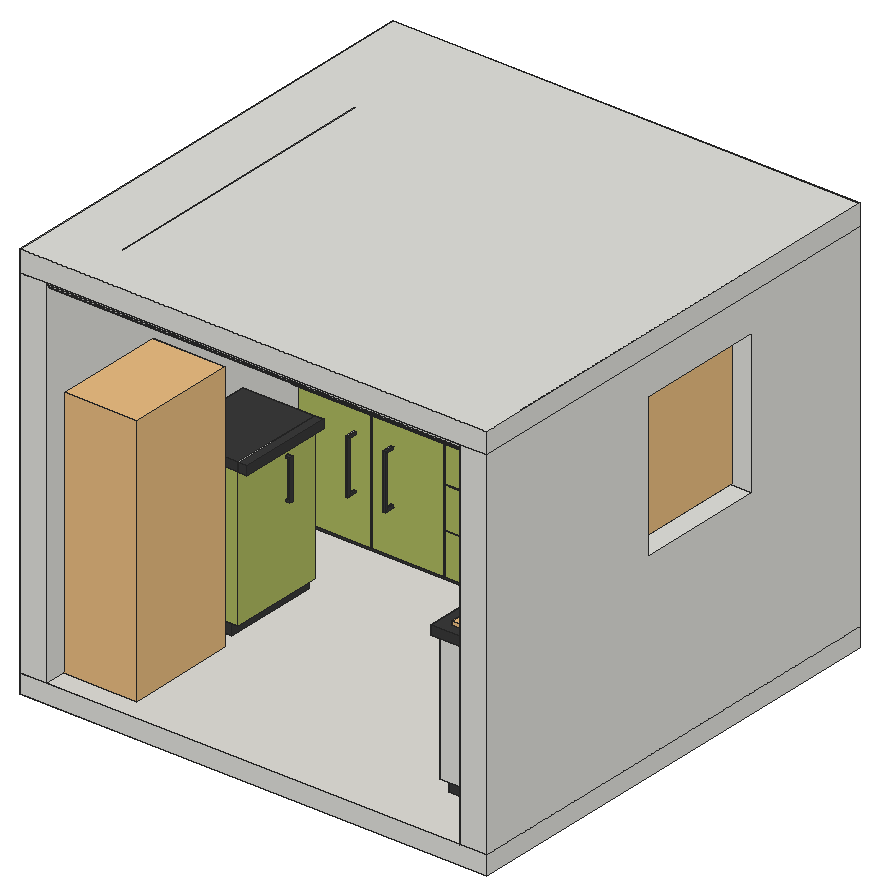
# SketchUp Ruby script. Lengths in inches.
U = 1.inch
M = Sketchup.active_model
def pt(a) = Geom::Point3d.new(a.map { |v| v * U })
def face(e, loops, mat)
  f = e.add_face(loops[0].map { |a| pt(a) })
  loops[1..].each { |l| e.add_face(l.map { |a| pt(a) }).erase! }
  f.material = f.back_material = mat if mat
  f
end
# faces: each face lists its corners as indices into pts; further lists are holes
def faces(e, pts, list, mat = nil) = list.each { |f| face(e, (f[0].is_a?(Array) ? f : [f]).map { |l| l.map { |i| pts[i] } }, mat) }
# xy, xz, yz: faces in a plane at the given z, y or x. An outline is a flat list of corners, or four numbers for a rectangle; further outlines are holes
def ring(l) = l.size == 4 ? [[l[0], l[1]], [l[2], l[1]], [l[2], l[3]], [l[0], l[3]]] : l.each_slice(2).to_a
def flat(e, list, mat, &to3) = list.each { |f| face(e, (f[0].is_a?(Array) ? f : [f]).map { |l| ring(l).map { |u, v| to3.(u, v) } }, mat) }
def xy(e, z, list, mat = nil) = flat(e, list, mat) { |x, y| [x, y, z] }
def xz(e, y, list, mat = nil) = flat(e, list, mat) { |x, z| [x, y, z] }
def yz(e, x, list, mat = nil) = flat(e, list, mat) { |y, z| [x, y, z] }
def lines(e, pts, list) = list.each { |a, b| e.add_line(pt(pts[a]), pt(pts[b])) }
# prism: a flat outline (further loops are holes) pulled along v
def prism(e, loops, v, mat = nil)
  f = face(e, loops, mat); d = Geom::Vector3d.new(v.map { |x| x * U })
  f.pushpull(f.normal.samedirection?(d) ? d.length : -d.length)
end
def box(e, o, s, mat = nil) = prism(e, [[o, [o[0] + s[0], o[1], o[2]], [o[0] + s[0], o[1] + s[1], o[2]], [o[0], o[1] + s[1], o[2]]]], [0, 0, s[2]], mat)
def at(x, y, z, deg = 0) = Geom::Transformation.translation(pt([x, y, z])) * Geom::Transformation.rotation(ORIGIN, Z_AXIS, deg.degrees)
def axes(o, x, y, z) = Geom::Transformation.new([*x, 0, *y, 0, *z, 0, *pt(o).to_a, 1])
def part(name) = M.definitions.add(name)
# library, detail: a bought-in or finely detailed component or shape, given as its bounding box
def library(name, o, s) = part(name).tap { |d| box(d.entities, o, s) }
def detail(e, o, s) = box(e.add_group.entities, o, s)
def put(e, d, t, mat = nil) = e.add_instance(d, t).tap { |i| i.material = mat if mat }
def group(e, t, mat = nil) = e.add_group.tap { |g| g.transformation = t; g.material = mat if mat }.entities
root = M.entities
M.materials.add("Decor - Olives").color = [174, 186, 96]
M.materials.add("[Color_007]").color = [58, 58, 58]
M.materials.add("[Marble Carrara Gold Floor Tile]").color = [225, 223, 217]
M.materials.add("[Tile Limestone Large]").color = [238, 251, 230]
M.materials.add("[Translucent Glass Dark Green]").color = [62, 91, 5]
M.materials["[Translucent Glass Dark Green]"].alpha = 0.5
M.materials.add("besi putih_Glossy3").color = [240, 240, 240]
M.materials.add("go trang").color = [128, 128, 128]
M.materials.add("sink-modena").color = [184, 184, 183]
c1 = library("Chimney (1)",[0,-14.34,0],[33.95,14.34,33.72])
c2 = library("365+Glass+Boxes",[-18.57,-9.91,0],[15.17,6.51,15.85])
c3 = library("FF_ceramic_large_dish_green_FMH",[0,0,0],[11.8125,11.8125,0.53])
c4 = library("FF_ceramic_medium_dish_blue_FMH",[0,0,0],[8.27,8.27,0.53])
c5 = library("FF_dish_rack_plastic_base_03_FMH",[-0.59,0,0],[11.88,20.6,0.91])
c6 = library("FF_dish_rack_cup_FMH\#1",[0,0.11,-0.46],[7.68,3.36,4.07])
c7 = library("FF_dish_rack_03_FMH",[0,0,0],[17.32,9.65,4.94])
c8 = library("FF_ceramic_medium_dish_red_FMH",[0,0,0],[8.27,8.27,0.53])
c9 = library("Kitchen utensil rack",[7.875,0,-1.06],[35.44,4.85,11.83])
c10 = library("kitchen",[57.57,5.21,10.61],[18.31,18.31,13.72])
c11 = library("French glass door with glass lintels",[-8.63,0,-6],[91.05,103.25,8])
c12 = library("Gas+stove+1",[-1.375,6.69,0.47],[35.625,31.32,3.01])
c13 = library("FF_flatware_wood_grip_placed_FMH\#1",[-5.7,-0.44,-1.47],[7.04,11.15,5.13])
c14 = library("Kitchen kettle",[-1.02,0.04,0],[9.81,8.74,8.22])
c15 = library("Drip coffee maker",[0,0,0.5],[20.95,10.01,8.67])
c16 = library("FF_Model_ID12346_3_IlluminatedPlanterCollectionLiscioCF3SU7",[0,0,0],[43.54,41.82,102.67])
c17 = library("itchenFaucet_Handspray\#1",[0.83,4.01,0],[10.6,4,15.3])
c18 = library("Kitchen towel rack",[0,0,-11.5625],[20.09,4.25,16.29])
c19 = library("Untitled (6)",[-101.41,0,-4.6],[35.6,35.6,49.16])
c20 = library("Component\#33",[0,0,0],[60.64,55.48,158.625])
c21 = library("Group\#225",[0,0,0],[3.9375,3.9375,5.51])
c22 = library("Group\#125",[0,0,-0.51],[31.38,18.97,5.43])
xy(root,-6.32,[[0,0,156.125,156.125]])
xy(root,0,[[0,0,0,156.125,156.125,156.125,156.125,0,147.125,0,147.125,20.1875,127.25,20.1875,127.25,108.125,9,108.125,9,81.875,31,81.875,31,50,9,50,9,0]])
xy(root,0,[[9,0,147.125,0,147.125,20.1875,127.25,20.1875,127.25,108.125,9,108.125,9,81.875,31,81.875,31,50,9,50]],"[Marble Carrara Gold Floor Tile]")
xy(root,3,[[124.25,20.1875,127.25,41.12],[124.55,41.12,127.25,41.42],[124.25,41.42,127.25,62.36],[124.55,62.36,127.25,62.66],[124.25,62.66,127.25,83.59],
  [124.55,83.59,127.25,83.89],[124.25,83.89,127.25,105.125],[9,105.125,33.4375,108.125],[33.74,105.125,33.74,105.43,33.4375,105.43,33.4375,108.125,57.875,108.125,57.875,105.125],[58.18,105.125,58.18,105.43,57.875,105.43,57.875,108.125,96.1875,108.125,96.1875,105.125],
  [96.49,105.125,96.49,105.43,96.1875,105.43,96.1875,108.125,127.25,108.125,127.25,105.125]])
xy(root,3.6875,[[9,50,31,81.875],[31,50,33,81.875]])
xy(root,7.66,[[69.52,103.2,69.52,105.125,70.21,105.125,70.21,103.88,79.5625,103.88,79.5625,105.125,80.25,105.125,80.25,103.2]],"[Color_007]")
xy(root,8.22,[[69.52,103.2,80.25,103.2,80.25,105.125,79.5625,105.125,79.5625,103.88,70.21,103.88,70.21,105.125,69.52,105.125]],"[Color_007]")
xy(root,16.7,[[58.18,105.125,96.1875,105.43]])
xy(root,17,[[58.18,105.125,96.1875,105.43]])
xy(root,23.22,[[69.52,103.2,69.52,105.125,70.21,105.125,70.21,103.88,79.5625,103.88,79.5625,105.125,80.25,105.125,80.25,103.2]],"[Color_007]")
xy(root,23.78,[[69.52,103.2,80.25,103.2,80.25,105.125,79.5625,105.125,79.5625,103.88,70.21,103.88,70.21,105.125,69.52,105.125]],"[Color_007]")
xy(root,30.7,[[58.18,105.125,96.1875,105.43]])
xy(root,31,[[58.18,105.125,96.1875,105.43]])
xy(root,38.78,[[69.52,103.2,69.52,105.125,70.21,105.125,70.21,103.88,79.5625,103.88,79.5625,105.125,80.25,105.125,80.25,103.2]],"[Color_007]")
xy(root,39.34,[[69.52,103.2,80.25,103.2,80.25,105.125,79.5625,105.125,79.5625,103.88,70.21,103.88,70.21,105.125,69.52,105.125]],"[Color_007]")
xy(root,41.75,[[127.45,24.52,143.57,57.2]])
xy(root,45,[[121.25,20.1875,124.25,41.12],[121.25,41.12,124.55,41.42],[121.25,41.42,124.25,62.36],[121.25,62.36,124.55,62.66],[121.25,62.66,124.25,83.59],
  [121.25,83.59,124.55,83.89],[121.25,83.89,124.25,102.125],[9,102.125,33.4375,105.125],[33.4375,102.125,33.74,105.43],[33.74,102.125,57.875,105.125],
  [57.875,102.125,58.18,105.43],[58.18,102.125,96.1875,105.125],[96.1875,102.125,96.49,105.43],[96.49,102.125,124.25,105.125]])
xy(root,48,[[[121.25,20.1875,147.125,20.1875,147.125,147.125,9,147.125,9,102.125,121.25,102.125],[127.45,24.52,143.57,57.2]]],"[Color_007]")
xy(root,49.75,[[33,50,36,81.875]])
xy(root,52.75,[[9,50,33,81.875],[33,50,36,81.875]],"[Color_007]")
xy(root,60,[[147.125,67.5625,156.125,111.125]])
xy(root,68.7,[[12,147.125,12.3,147.43],[12.3,147.125,38.43,147.43],[38.43,147.125,38.73,147.43],[38.73,147.125,64.85,147.43],[64.85,147.125,65.15,147.43],
  [117.7,147.125,118,147.43],[118,147.125,144.125,147.43]])
xy(root,69,[[12.3,123.125,38.43,147.43],[38.73,123.125,64.85,147.43],[118,123.125,144.125,147.43],[144.43,123.125,144.43,123.43,144.125,123.43,144.125,147.125,147.125,147.125,147.125,123.125]])
xy(root,71.38,[[121.15,122.4375,139,123.125]])
xy(root,71.68,[[43.32,122.5,60.58,123.125]])
xy(root,72.4,[[122.17,122.4375,137.98,123.125],[44.04,122.5,59.86,123.125]])
xy(root,72.74,[[34.72,121.68,35.28,123.125],[40.84,121.68,41.41,123.125],[140.37,121.68,140.93,123.125]])
xy(root,73.42,[[34.69,122.37,35.25,123.125],[40.82,122.37,41.38,123.125],[140.34,122.37,140.9,123.125]],"[Color_007]")
xy(root,82,[[34.69,122.37,35.25,123.125],[40.82,122.37,41.38,123.125],[140.34,122.37,140.9,123.125]])
xy(root,82.69,[[34.72,121.68,35.28,123.125],[40.84,121.68,41.41,123.125],[140.37,121.68,140.93,123.125]],"[Color_007]")
xy(root,89.21,[[122.17,122.4375,137.98,123.125],[44.04,122.5,59.86,123.125]])
xy(root,89.93,[[43.32,122.5,60.58,123.125]])
xy(root,90.23,[[121.15,122.4375,139,123.125]])
xy(root,92.7,[[12.3,123.125,38.43,147.43],[38.73,123.125,64.85,147.43],[118,123.125,144.125,147.43],[144.125,123.43,144.43,147.43],[65.15,147.125,117.7,147.43]])
xy(root,93,[[12.3,123.125,38.43,147.43],[38.73,123.125,64.85,147.43],[65.15,123.125,91.28,147.43],[91.58,123.125,117.7,147.43],[118,123.125,144.125,147.43],
  [144.125,123.51,144.43,147.125],[144.125,147.125,144.43,147.43]])
xy(root,95.74,[[34.72,121.68,35.28,123.125]])
xy(root,96.18,[[41.59,121.68,42.15,123.125],[87.4,121.68,87.96,123.125],[94.34,121.68,94.9,123.125],[140.37,121.68,140.93,123.125]])
xy(root,96.42,[[34.69,122.37,35.25,123.125]],"[Color_007]")
xy(root,96.86,[[41.56,122.37,42.12,123.125],[87.37,122.37,87.93,123.125],[94.31,122.37,94.87,123.125],[140.34,122.37,140.9,123.125]],"[Color_007]")
xy(root,105,[[34.69,122.37,35.25,123.125]])
xy(root,105.44,[[41.56,122.37,42.12,123.125],[87.37,122.37,87.93,123.125],[94.31,122.37,94.87,123.125],[140.34,122.37,140.9,123.125]])
xy(root,105.69,[[34.72,121.68,35.28,123.125]],"[Color_007]")
xy(root,106.13,[[41.59,121.68,42.15,123.125],[87.4,121.68,87.96,123.125],[94.34,121.68,94.9,123.125],[140.37,121.68,140.93,123.125]],"[Color_007]")
xy(root,108,[[147.125,67.5625,156.125,111.125]])
xy(root,117,[[12,147.125,12.3,147.43],[12.3,147.125,38.43,147.43],[38.43,147.125,38.73,147.43],[38.73,147.125,64.85,147.43],[64.85,147.125,65.15,147.43],
  [65.15,147.125,91.28,147.43],[91.28,147.125,91.58,147.43],[91.58,147.125,117.7,147.43],[117.7,147.125,118,147.43],[118,147.125,144.125,147.43]])
xy(root,120,[[0,0,0,156.125,156.125,156.125,156.125,0,147.125,0,147.125,147.125,144.125,147.125,144.125,147.43,118,147.43,118,147.125,117.7,147.125,117.7,147.43,91.58,147.43,91.58,147.125,91.28,147.125,91.28,147.43,65.15,147.43,65.15,147.125,64.85,147.125,64.85,147.43,38.73,147.43,38.73,147.125,38.43,147.125,38.43,147.43,12.3,147.43,12.3,147.125,9,147.125,9,0],[12.3,3.3,12.3,123.125,12.63,123.125,12.63,3.63,143.49,3.63,143.82,46.28,143.82,3.3],[[12.63,3.63,12.63,123.125,12.3,123.125,12.3,147.125,38.43,147.125,38.43,143.49,38.73,143.49,38.73,123.125,64.85,123.125,64.85,143.49,65.15,143.49,65.15,123.125,91.28,123.125,91.28,143.49,91.58,143.49,91.58,147.125,117.7,147.125,117.7,123.125,144.43,123.125,144.33,121,143.83,121,143.82,46.28,143.49,3.63],[12.63,123.125,38.43,123.125,38.43,143.49,34.79,143.49,34.79,143.79,15.93,143.79,15.93,143.49,12.63,143.49],[91.58,123.125,114.37,123.125,114.37,143.49,114.07,143.49,114.07,143.79,95.21,143.79,95.21,143.49,91.58,143.49]],[144.33,121,144.43,123.125,147.125,123.125,147.125,121],[12.3,123.125,12.63,123.125,12.63,143.49,15.93,143.49,15.93,143.79,34.79,143.79,34.79,143.49,38.43,143.49,38.43,147.125,12.3,147.125],
  [12.63,123.125,12.63,143.49,15.93,143.49,15.93,143.79,34.79,143.79,34.79,143.49,38.43,143.49,38.43,123.125],[38.73,123.125,38.73,143.49,42.36,143.49,42.36,143.79,61.22,143.79,61.22,143.49,64.85,143.49,64.85,123.125],[65.15,123.125,65.15,143.49,68.78,143.49,68.78,143.79,87.64,143.79,87.64,143.49,91.28,143.49,91.28,123.125],[91.58,123.125,91.58,143.49,95.21,143.49,95.21,143.79,114.07,143.79,114.07,143.49,114.37,143.49,114.37,123.125],[117.7,123.125,118,147.125],
  [118,123.125,144.125,147.125],[144.125,123.125,144.43,123.51],[144.43,123.125,144.43,123.51,144.125,123.51,144.125,147.125,147.125,147.125,147.125,123.125],[9,125.4,12.3,147.125],[38.43,143.49,38.73,147.125],
  [38.73,143.49,38.73,147.125,64.85,147.125,64.85,143.49,61.22,143.49,61.22,143.79,42.36,143.79,42.36,143.49],[64.85,143.49,65.15,147.125],[65.15,143.49,65.15,147.125,91.28,147.125,91.28,143.49,87.64,143.49,87.64,143.79,68.78,143.79,68.78,143.49],[91.28,143.49,91.58,147.125],[12.3,147.125,38.43,147.43],
  [38.73,147.125,64.85,147.43],[38.73,147.125,64.85,147.43],[65.15,147.125,91.28,147.43],[65.15,147.125,91.28,147.43],[91.58,147.125,117.7,147.43],
  [118,147.125,144.125,147.43]])
xy(root,127.14,[[0,0,156.125,156.125]])
xz(root,0,[[0,-6.32,156.125,0],[0,0,9,120],[147.125,0,156.125,120],[0,120,156.125,127.14]])
xz(root,20.1875,[[124.25,3,147.125,45]])
xz(root,20.1875,[[127.25,0,147.125,3],[121.25,45,147.125,48]],"[Color_007]")
xz(root,24.52,[[127.45,41.75,143.57,48]])
xz(root,41.12,[[124.25,3,124.55,45]])
xz(root,41.42,[[124.25,3,124.55,45]])
xz(root,50,[[9,3.6875,33,49.75]],"Decor - Olives")
xz(root,50,[[9,0,31,3.6875],[9,49.75,33,52.75],[33,49.75,36,52.75]],"[Color_007]")
xz(root,57.2,[[127.45,41.75,143.57,48]])
xz(root,62.36,[[124.25,3,124.55,45]])
xz(root,62.66,[[124.25,3,124.55,45]])
xz(root,67.5625,[[147.125,60,156.125,108]])
xz(root,69.62,[[32.25,32.39,34.66,32.39,34.66,46.14,33,46.14,33,45.33,33.84,45.33,33.84,33.2,32.25,33.2]],"[Color_007]")
xz(root,70.63,[[32.25,32.38,32.25,33.19,33.85,33.19,33.85,45.34,33,45.34,33,46.15,34.67,46.15,34.67,32.38]],"[Color_007]")
xz(root,81.875,[[9,0,31,3.6875],[9,3.6875,33,52.75],[33,49.75,36,52.75]])
xz(root,83.59,[[124.25,3,124.55,45]])
xz(root,83.89,[[124.25,3,124.55,45]])
xz(root,102.125,[[9,45,121.25,48]],"[Color_007]")
xz(root,103.2,[[69.52,7.66,80.25,8.22],[69.52,23.22,80.25,23.78],[69.52,38.78,80.25,39.34]],"[Color_007]")
xz(root,103.88,[[70.21,7.66,79.5625,8.22],[70.21,23.22,79.5625,23.78],[70.21,38.78,79.5625,39.34]])
xz(root,105.125,[[27.53,35.13,27.54,35.9,28.36,35.92,28.35,35.14],[69.52,38.78,70.21,39.34]])
xz(root,105.125,[[[9,3,33.4375,45],[28.36,17.6,27.54,17.62,27.53,18.39,28.35,18.375],[27.53,35.13,27.54,35.9,28.36,35.92,28.35,35.14]],[33.74,3,57.875,45],[58.18,3,96.1875,16.7],[96.49,3,124.25,45],[58.18,17,96.1875,30.7],
  [[58.18,31,96.1875,45],[69.52,38.78,70.21,39.34],[79.5625,38.78,80.25,39.34]]],"Decor - Olives")
xz(root,105.43,[[33.4375,3,33.74,45],[57.875,3,58.18,16.7],[96.1875,3,96.49,45],[57.875,16.7,96.1875,17],[57.875,17,58.18,17,58.18,30.7,96.1875,30.7,96.1875,31,58.18,31,58.18,45,57.875,45]])
xz(root,108.125,[[9,0,127.25,3]],"[Color_007]")
xz(root,111.125,[[147.125,60,156.125,108]])
xz(root,121,[[145.48,117.99,145.05,118.0625,144.65,118.26,144.31,118.58,144.05,119,143.88,119.48,143.83,120,147.125,120,147.07,119.48,146.9,119,146.64,118.58,146.3,118.26,145.9,118.0625]])
xz(root,121.68,[[34.72,72.74,35.28,82.69],[40.84,72.74,41.41,82.69],[140.37,72.74,140.93,82.69],[34.72,95.74,35.28,105.69],[41.59,96.18,42.15,106.13],
  [87.4,96.18,87.96,106.13],[94.34,96.18,94.9,106.13],[140.37,96.18,140.93,106.13]],"[Color_007]")
xz(root,122.37,[[34.69,73.42,35.25,82],[40.82,73.42,41.38,82],[140.34,73.42,140.9,82],[34.69,96.42,35.25,105],[41.56,96.86,42.12,105.44],
  [87.37,96.86,87.93,105.44],[94.31,96.86,94.87,105.44],[140.34,96.86,140.9,105.44]])
xz(root,122.4375,[[[121.15,71.38,139,90.23],[122.17,72.4,137.98,89.21]]])
xz(root,122.5,[[[43.32,71.68,60.58,89.93],[44.04,72.4,59.86,89.21]]])
xz(root,123.125,[[12.3,69,38.43,92.7],[[38.73,69,64.85,92.7],[43.32,71.68,60.58,89.93]],[[118,69,144.125,92.7],[121.15,71.38,139,90.23]],[144.43,69,147.125,93],[12.3,93,38.43,120],
  [38.73,93,64.85,120],[65.15,93,91.28,120],[91.58,93,117.7,120],[118,93,144.125,120],[144.43,93,147.125,120]])
xz(root,123.125,[[44.04,72.4,59.86,89.21],[122.17,72.4,137.98,89.21]],"[Translucent Glass Dark Green]")
xz(root,123.43,[[144.125,69,144.43,92.7]])
xz(root,123.51,[[144.125,93,144.43,120]])
xz(root,125.4,[[10.65,117.99,10.22,118.0625,9.83,118.26,9.48,118.58,9.22,119,9.06,119.48,9,120,12.3,120,12.24,119.48,12.08,119,11.82,118.58,11.47,118.26,11.08,118.0625]])
xz(root,147.125,[[9,69,12,93],[9,93,12,117],[9,117,144.125,120]])
xz(root,147.125,[[9,48,147.125,48,147.125,69,144.125,69,144.125,68.7,117.7,68.7,117.7,69,65.15,69,65.15,68.7,12,68.7,12,69,9,69],[65.15,69,117.7,92.7]],"[Tile Limestone Large]")
xz(root,147.43,[[12,68.7,65.15,69],[117.7,68.7,144.125,69],[12,69,12.3,69,12.3,92.7,38.43,92.7,38.43,69,38.73,69,38.73,92.7,64.85,92.7,64.85,69,65.15,69,65.15,92.7,117.7,92.7,117.7,69,118,69,118,92.7,144.43,92.7,144.43,93,118,93,118,117,117.7,117,117.7,93,91.58,93,91.58,117,91.28,117,91.28,93,65.15,93,65.15,117,64.85,117,64.85,93,38.73,93,38.73,117,38.43,117,38.43,93,12.3,93,12.3,117,12,117],[12.3,117,38.43,120],[38.73,117,64.85,120],
  [65.15,117,91.28,120],[91.58,117,117.7,120],[118,117,144.125,120]])
xz(root,156.125,[[0,-6.32,156.125,0],[0,0,156.125,120],[0,120,156.125,127.14]])
yz(root,0,[[0,-6.32,156.125,0],[0,0,156.125,120],[0,120,156.125,127.14]])
yz(root,9,[[0,0,50,0,50,52.75,81.875,52.75,81.875,0,108.125,0,108.125,3,105.125,3,105.125,45,102.125,45,102.125,48,147.125,48,147.125,120,0,120],[50,3.6875,81.875,52.75]])
yz(root,12,[[147.125,68.7,147.43,69],[147.125,69,147.43,93],[147.125,93,147.43,117]])
yz(root,12.3,[[123.125,69,147.43,92.7],[123.125,93,147.43,120]])
yz(root,31,[[50,0,81.875,3.6875]],"[Color_007]")
yz(root,32.25,[[70.63,32.38,69.62,32.39,69.62,33.2,70.63,33.19]],"Decor - Olives")
yz(root,33,[[50,49.75,81.875,52.75]])
yz(root,33,[[[50,3.6875,81.875,49.75],[69.62,45.33,69.62,46.14,70.63,46.15,70.63,45.34]],[69.62,45.33,69.62,46.14,70.63,46.15,70.63,45.34]],"Decor - Olives")
yz(root,33.4375,[[105.125,3,105.43,45]])
yz(root,33.74,[[105.125,3,105.43,45]])
yz(root,36,[[50,49.75,81.875,52.75]],"[Color_007]")
yz(root,38.43,[[123.125,69,147.43,92.7],[123.125,93,147.43,120]])
yz(root,38.73,[[123.125,69,147.43,92.7],[123.125,93,147.43,120]])
yz(root,43.32,[[122.5,71.68,123.125,89.93]])
yz(root,44.04,[[122.5,72.4,123.125,89.21]])
yz(root,57.875,[[105.125,3,105.43,16.7],[105.125,16.7,105.43,17],[105.125,17,105.43,45]])
yz(root,58.18,[[105.125,3,105.43,16.7],[105.125,17,105.43,30.7],[105.125,31,105.43,45]])
yz(root,59.86,[[122.5,72.4,123.125,89.21]])
yz(root,60.58,[[122.5,71.68,123.125,89.93]])
yz(root,64.85,[[123.125,69,147.43,92.7],[123.125,93,147.43,120]])
yz(root,65.15,[[147.125,68.7,147.43,69],[147.125,69,147.43,92.7],[123.125,93,147.43,120]])
yz(root,69.52,[[103.2,7.66,105.125,8.22],[103.2,23.22,105.125,23.78],[103.2,38.78,105.125,39.34]],"[Color_007]")
yz(root,70.21,[[103.88,7.66,105.125,8.22],[103.88,23.22,105.125,23.78],[103.88,38.78,105.125,39.34]],"[Color_007]")
yz(root,79.5625,[[103.88,7.66,105.125,8.22],[103.88,23.22,105.125,23.78],[103.88,38.78,105.125,39.34]],"[Color_007]")
yz(root,80.25,[[103.2,7.66,105.125,8.22],[103.2,23.22,105.125,23.78],[103.2,38.78,105.125,39.34]],"[Color_007]")
yz(root,91.28,[[123.125,93,147.43,120]])
yz(root,91.58,[[123.125,93,147.43,120]])
yz(root,96.1875,[[105.125,3,105.43,16.7],[105.125,17,105.43,30.7],[105.125,31,105.43,45]])
yz(root,96.49,[[105.125,3,105.43,16.7],[105.125,16.7,105.43,17],[105.125,17,105.43,30.7],[105.125,30.7,105.43,31],[105.125,31,105.43,45]])
yz(root,101.64,[[101.83,17.62,101.83,35.9,102.6,35.13,102.6,18.39],[101.83,17.62,102.6,18.39,105.125,18.39,105.125,17.62],[102.6,35.13,101.83,35.9,105.125,35.9,105.125,35.13]],"[Color_007]")
yz(root,102.46,[[101.8125,17.6,102.59,18.375,102.59,35.14,101.8125,35.92],[101.8125,17.6,105.125,17.6,105.125,18.375,102.59,18.375],[102.59,35.14,105.125,35.14,105.125,35.92,101.8125,35.92]],"[Color_007]")
yz(root,117.7,[[147.125,68.7,147.43,69],[147.125,69,147.43,69.375],[147.125,69.375,147.43,92.7],[123.125,93,147.43,93.375],[123.125,93.375,147.43,120]])
yz(root,118,[[123.125,69,147.43,69.375],[123.125,69.375,147.43,92.7],[123.125,93,147.43,93.375],[123.125,93.375,147.43,120]])
yz(root,121.15,[[122.4375,71.38,123.125,90.23]])
yz(root,121.25,[[20.1875,45,102.125,48]],"[Color_007]")
yz(root,122.17,[[122.4375,72.4,123.125,89.21]])
yz(root,124.25,[[88.3,34.44,88.35,35.3125,87.59,35.34,87.55,34.46]])
yz(root,124.25,[[20.1875,3,41.12,45],[41.42,3,62.36,45],[62.66,3,83.59,45],[[83.89,3,105.125,45],[87.59,17.1875,88.35,17.21,88.3,18.08,87.55,18.06],[88.3,34.44,88.35,35.3125,87.59,35.34,87.55,34.46]]],"Decor - Olives")
yz(root,124.55,[[41.12,3,41.42,45],[62.36,3,62.66,45],[83.59,3,83.89,45]])
yz(root,127.25,[[20.1875,0,108.125,3]],"[Color_007]")
yz(root,127.45,[[24.52,41.75,57.2,48]])
yz(root,137.98,[[122.4375,72.4,123.125,89.21]])
yz(root,139,[[122.4375,71.38,123.125,90.23]])
yz(root,143.57,[[24.52,41.75,57.2,48]])
yz(root,144.125,[[147.125,68.7,147.43,69],[123.125,69,123.43,92.7],[123.125,93,123.51,120],[123.51,93,123.51,120,147.125,120,147.125,117,147.43,117,147.43,93],[147.125,117,147.43,120]])
yz(root,144.43,[[123.125,69,123.43,92.7],[123.125,92.7,147.43,93],[123.125,93,123.51,120]])
yz(root,147.125,[[[0,0,0,120,123.125,120,123.125,69,147.125,69,147.125,48,20.1875,48,20.1875,0],[67.5625,60,111.125,108]]])
yz(root,156.125,[[0,-6.32,156.125,0],[[0,0,156.125,120],[67.5625,60,111.125,108]],[0,120,156.125,127.14]])
p = [[122.58,36.42,18.06],[121.71,36.47,17.1875],[124.25,36.47,17.1875],[124.25,36.42,18.06],[122.58,36.42,34.46],[121.71,36.47,35.34],
  [121.73,37.22,35.3125],[121.73,37.22,17.21],[122.61,37.18,18.08],[124.25,37.18,18.08],[124.25,37.22,17.21],[122.61,37.18,34.44],
  [122.58,43.74,34.46],[121.71,43.78,35.34],[121.71,43.78,17.1875],[122.58,43.74,18.06],[124.25,43.78,17.1875],[124.25,43.74,18.06],
  [121.73,44.54,35.3125],[121.73,44.54,17.21],[122.61,44.49,18.08],[124.25,44.49,18.08],[124.25,44.54,17.21],[122.61,44.49,34.44],
  [121.71,64.84,35.34],[121.73,65.6,35.3125],[121.73,65.6,17.21],[121.71,64.84,17.1875],[122.58,64.8,34.46],[122.58,64.8,18.06],
  [124.25,64.84,17.1875],[124.25,64.8,18.06],[122.61,65.55,18.08],[124.25,65.55,18.08],[124.25,65.6,17.21],[122.61,65.55,34.44],
  [122.58,87.55,34.46],[121.71,87.59,35.34],[121.71,87.59,17.1875],[122.58,87.55,18.06],[124.25,87.59,17.1875],[124.25,87.55,18.06],
  [121.73,88.35,35.3125],[121.73,88.35,17.21],[124.25,88.35,17.21],[122.61,88.3,34.44],[122.61,88.3,18.08],[124.25,88.3,18.08],
  [28.36,101.8125,17.6],[27.54,101.83,17.62],[27.54,105.125,17.62],[28.36,105.125,17.6],[27.53,102.6,18.39],[27.53,105.125,18.39],
  [27.54,101.83,35.9],[27.53,102.6,35.13],[28.36,101.8125,35.92],[28.35,102.59,18.375],[28.35,105.125,18.375],[28.35,102.59,35.14],
  [40.84,101.8125,17.6],[40.02,101.83,17.62],[40.02,105.125,17.62],[40.84,105.125,17.6],[40.01,102.6,18.39],[40.01,105.125,18.39],
  [40.84,101.8125,35.92],[40.02,101.83,35.9],[40.01,102.6,35.13],[40.83,102.59,35.14],[40.83,102.59,18.375],[40.83,105.125,18.375],
  [102.46,101.8125,35.92],[101.64,101.83,35.9],[101.64,101.83,17.62],[102.46,101.8125,17.6],[101.64,105.125,17.62],[102.46,105.125,17.6],
  [101.64,102.6,35.13],[102.46,102.59,35.14],[102.46,102.59,18.375],[101.64,102.6,18.39],[102.46,105.125,18.375],[101.64,105.125,18.39],
  [34.67,70.63,32.38],[34.66,69.62,32.39],[32.25,69.62,32.39],[32.25,70.63,32.38],[34.67,70.63,46.15],[34.66,69.62,46.14],
  [33.84,69.62,33.2],[33.85,70.63,33.19],[32.25,70.63,33.19],[32.25,69.62,33.2],[33.84,69.62,45.33],[33.85,70.63,45.34],
  [124.25,37.18,34.44],[124.25,36.42,34.46],[124.25,37.22,35.3125],[124.25,44.49,34.44],[124.25,43.74,34.46],[124.25,44.54,35.3125],
  [124.25,65.55,34.44],[124.25,64.8,34.46],[124.25,65.6,35.3125],[124.25,88.3,34.44],[124.25,87.55,34.46],[124.25,88.35,35.3125],
  [124.25,36.47,35.34],[124.25,43.78,35.34],[124.25,64.84,35.34],[124.25,87.59,35.34],[27.54,105.125,35.9],[27.53,105.125,35.13],
  [28.35,105.125,35.14],[28.36,105.125,35.92],[40.02,105.125,35.9],[40.01,105.125,35.13],[40.83,105.125,35.14],[40.84,105.125,35.92],
  [101.64,105.125,35.13],[102.46,105.125,35.14],[102.46,105.125,35.92],[101.64,105.125,35.9],[33,69.62,45.33],[33,70.63,45.34],
  [33,70.63,46.15],[33,69.62,46.14],[34.72,121.68,72.74],[34.69,122.37,73.42],[34.69,123.125,73.42],[34.72,123.125,72.74],
  [34.72,121.68,82.69],[34.69,122.37,82],[35.25,122.37,73.42],[35.28,121.68,72.74],[35.28,123.125,72.74],[35.25,123.125,73.42],
  [35.25,122.37,82],[35.28,121.68,82.69],[40.84,121.68,82.69],[40.82,122.37,82],[40.82,122.37,73.42],[40.84,121.68,72.74],
  [40.82,123.125,73.42],[40.84,123.125,72.74],[41.38,122.37,82],[41.41,121.68,82.69],[41.41,121.68,72.74],[41.38,122.37,73.42],
  [41.41,123.125,72.74],[41.38,123.125,73.42],[140.37,121.68,82.69],[140.34,122.37,82],[140.34,122.37,73.42],[140.37,121.68,72.74],
  [140.34,123.125,73.42],[140.37,123.125,72.74],[140.9,122.37,73.42],[140.93,121.68,72.74],[140.93,123.125,72.74],[140.9,123.125,73.42],
  [140.9,122.37,82],[140.93,121.68,82.69],[34.72,123.125,82.69],[34.69,123.125,82],[35.25,123.125,82],[35.28,123.125,82.69],
  [40.84,123.125,82.69],[40.82,123.125,82],[41.38,123.125,82],[41.41,123.125,82.69],[140.37,123.125,82.69],[140.34,123.125,82],
  [140.9,123.125,82],[140.93,123.125,82.69],[34.72,121.68,105.69],[34.69,122.37,105],[34.69,122.37,96.42],[34.72,121.68,95.74],
  [34.69,123.125,96.42],[34.72,123.125,95.74],[35.25,122.37,105],[35.28,121.68,105.69],[35.28,121.68,95.74],[35.25,122.37,96.42],
  [35.28,123.125,95.74],[35.25,123.125,96.42],[41.59,121.68,96.18],[41.56,122.37,96.86],[41.56,123.125,96.86],[41.59,123.125,96.18],
  [41.59,121.68,106.13],[41.56,122.37,105.44],[42.12,122.37,105.44],[42.15,121.68,106.13],[42.15,121.68,96.18],[42.12,122.37,96.86],
  [42.15,123.125,96.18],[42.12,123.125,96.86],[87.4,121.68,96.18],[87.37,122.37,96.86],[87.37,123.125,96.86],[87.4,123.125,96.18],
  [87.4,121.68,106.13],[87.37,122.37,105.44],[87.93,122.37,96.86],[87.96,121.68,96.18],[87.96,123.125,96.18],[87.93,123.125,96.86],
  [87.93,122.37,105.44],[87.96,121.68,106.13],[94.34,121.68,96.18],[94.31,122.37,96.86],[94.31,123.125,96.86],[94.34,123.125,96.18],
  [94.34,121.68,106.13],[94.31,122.37,105.44],[94.87,122.37,96.86],[94.9,121.68,96.18],[94.9,123.125,96.18],[94.87,123.125,96.86],
  [94.87,122.37,105.44],[94.9,121.68,106.13],[140.37,121.68,106.13],[140.34,122.37,105.44],[140.34,122.37,96.86],[140.37,121.68,96.18],
  [140.34,123.125,96.86],[140.37,123.125,96.18],[140.9,122.37,96.86],[140.93,121.68,96.18],[140.93,123.125,96.18],[140.9,123.125,96.86],
  [140.9,122.37,105.44],[140.93,121.68,106.13],[34.72,123.125,105.69],[34.69,123.125,105],[35.25,123.125,105],[35.28,123.125,105.69],
  [41.59,123.125,106.13],[41.56,123.125,105.44],[42.12,123.125,105.44],[42.15,123.125,106.13],[87.4,123.125,106.13],[87.37,123.125,105.44],
  [87.93,123.125,105.44],[87.96,123.125,106.13],[94.34,123.125,106.13],[94.31,123.125,105.44],[94.87,123.125,105.44],[94.9,123.125,106.13],
  [140.37,123.125,106.13],[140.34,123.125,105.44],[140.9,123.125,105.44],[140.93,123.125,106.13],[10.22,125.4,118.0625],[10.65,125.4,117.99],
  [10.65,1.65,117.99],[10.22,1.22,118.0625],[145.47,1.65,117.99],[145.9,1.22,118.0625],[145.48,121,117.99],[145.9,121,118.0625],
  [11.08,125.4,118.0625],[11.08,2.08,118.0625],[145.05,2.08,118.0625],[145.05,121,118.0625],[9.83,125.4,118.26],[9.82,0.83,118.26],
  [146.3,0.83,118.26],[146.3,121,118.26],[11.47,125.4,118.26],[11.47,2.48,118.26],[144.65,2.48,118.26],[144.65,121,118.26],
  [9.48,125.4,118.58],[9.48,0.48,118.58],[146.64,0.48,118.58],[146.64,121,118.58],[11.82,125.4,118.58],[11.82,2.82,118.58],
  [144.31,2.82,118.58],[144.31,121,118.58],[9.22,125.4,119],[9.22,0.22,119],[146.9,0.22,119],[146.9,121,119],
  [12.08,125.4,119],[12.08,3.08,119],[144.05,3.08,119],[144.05,121,119],[9.06,125.4,119.48],[9.06,0.06,119.48],
  [147.07,0.06,119.48],[147.07,121,119.48],[12.24,125.4,119.48],[12.24,3.24,119.48],[143.88,3.24,119.48],[143.88,121,119.48],
  [9,125.4,120],[9,0,120],[147.125,0,120],[147.125,121,120],[12.3,125.4,120],[12.3,123.125,120],
  [12.3,3.3,120],[143.82,3.3,120],[143.82,46.28,120],[143.83,121,120],[69.88,103.5625,39.12],[79.88,103.5625,39.12],
  [79.88,105.125,39.12],[69.88,105.125,39.12],[122.125,87.81,34.92],[122.125,87.81,17.6],[28.08,102.125,35.6],[28.08,102.125,17.91],
  [28.08,105.125,17.91],[124.25,87.81,34.92],[28.08,105.125,35.6],[124.25,87.81,17.6],[826.26,232.85,133.86],[834.9,232.85,133.86],
  [834.9,277.98,133.86],[826.26,251.3,133.86],[33,69.97,45.86],[34.375,69.97,45.86],[34.375,69.97,32.67],[32.25,69.97,32.67]]
faces(root,p,[[0,1,2,3],[4,5,1,0],[5,6,7,1],[7,8,9,10],[6,11,8,7],[12,13,14,15],[15,14,16,17],[13,18,19,14],
  [19,20,21,22],[18,23,20,19],[24,25,26,27],[28,24,27,29],[29,27,30,31],[26,32,33,34],[25,35,32,26],[36,37,38,39],
  [39,38,40,41],[37,42,43,38],[42,45,46,43],[43,46,47,44],[48,49,50,51],[56,54,49,48],[57,48,51,58],[59,56,48,57],
  [60,61,62,63],[61,64,65,62],[66,67,61,60],[67,68,64,61],[69,66,60,70],[70,60,63,71],[72,73,74,75],[8,0,3,9],
  [20,15,17,21],[32,29,31,33],[46,39,41,47],[52,57,58,53],[64,70,71,65],[81,80,82,83],[84,85,86,87],[88,89,85,84],
  [90,91,92,93],[98,96,11,6],[99,100,12,23],[101,99,23,18],[104,102,35,25],[107,105,45,42],[97,108,5,4],[100,109,13,12],
  [103,110,24,28],[106,111,37,36],[114,115,56,59],[118,119,66,69],[120,121,79,78],[108,98,6,5],[109,101,18,13],[110,104,25,24],
  [111,107,42,37],[115,112,54,56],[119,116,67,66],[122,123,73,72],[126,127,89,88],[128,129,130,131],[132,133,129,128],[134,135,136,137],
  [138,139,135,134],[140,141,142,143],[143,142,144,145],[146,147,148,149],[149,148,150,151],[152,153,154,155],[155,154,156,157],[158,159,160,161],
  [162,163,159,158],[164,165,133,132],[166,167,139,138],[168,169,141,140],[170,171,147,146],[172,173,153,152],[174,175,163,162],[176,177,178,179],
  [179,178,180,181],[182,183,184,185],[185,184,186,187],[188,189,190,191],[192,193,189,188],[194,195,196,197],[197,196,198,199],[200,201,202,203],
  [204,205,201,200],[206,207,208,209],[210,211,207,206],[212,213,214,215],[216,217,213,212],[218,219,220,221],[222,223,219,218],[224,225,226,227],
  [227,226,228,229],[230,231,232,233],[234,235,231,230],[236,237,177,176],[238,239,183,182],[240,241,193,192],[242,243,195,194],[244,245,205,204],
  [246,247,211,210],[248,249,217,216],[250,251,223,222],[252,253,225,224],[254,255,235,234]],"[Color_007]")
faces(root,p,[[38,43,44,40],[49,52,53,50],[54,55,52,49],[75,74,76,77],[11,4,0,8],[23,12,15,20],[35,28,29,32],[45,36,39,46],
  [55,59,57,52],[68,69,70,64],[78,79,80,81],[96,97,4,11],[102,103,28,35],[105,106,36,45],[112,113,55,54],[116,117,68,67],
  [113,114,59,55],[117,118,69,68],[256,257,258,259],[259,258,260,261],[261,260,262,263],[257,264,265,258],[258,265,266,260],[260,266,267,262],
  [268,256,259,269],[269,259,261,270],[270,261,263,271],[264,272,273,265],[265,273,274,266],[266,274,275,267],[276,268,269,277],[277,269,270,278],
  [278,270,271,279],[272,280,281,273],[273,281,282,274],[274,282,283,275],[284,276,277,285],[285,277,278,286],[286,278,279,287],[280,288,289,281],
  [281,289,290,282],[282,290,291,283],[292,284,285,293],[293,285,286,294],[294,286,287,295],[288,296,297,289],[289,297,298,290],[290,298,299,291],
  [300,292,293,301],[301,293,294,302],[302,294,295,303],[296,304,305,306,297],[297,306,307,298],[298,307,308,309,299]])
faces(root,p,[[94,95,91,90],[124,125,95,94]],"Decor - Olives")
lines(root,p,[[310,311],[311,312],[313,310],[314,315],[316,317],[317,318],[319,314],[320,316],[315,321],[322,323],[323,324],[325,322],
  [326,327],[327,328],[328,329]])
put(root,c1,axes([74.03,132.75,68.98],[1.0602,0,0],[0,0.93,0],[0,0,0.93]))
put(root,c2,axes([64.71,138.9375,72.2],[0.96,0,0],[0,0.96,0],[0,0,0.8544]))
put(root,c2,axes([56.96,138.9375,72.2],[0.96,0,0],[0,0.96,0],[0,0,0.8544]))
put(root,c3,axes([52.2,140.5,62.11],[-0.26351,0,-1.0782],[0,-1.1027,0],[-1.22915,0,0.23115]),"go trang")
put(root,c4,axes([45.57,128.92,59.36],[-0.32844,0,-1.19087],[0,1.22522,0],[1.35759,0,-0.2881]),"go trang")
put(root,c5,axes([31.19,140.54,48.1],[0,-1.22522,0],[1.39676,0,0],[0,0,1.22522]),"go trang")
put(root,c6,axes([56.68,129.14,49.87],[0,1.22522,0],[-1.39676,0,0],[0,0,1.22522]),"go trang")
put(root,c7,axes([33.55,128.08,48.2],[1.39676,0,0],[0,1.22522,0],[0,0,1.22522]),"go trang")
put(root,c8,axes([46.875,128.92,59.36],[-0.32844,0,-1.19087],[0,1.22522,0],[1.35759,0,-0.2881]),"go trang")
put(root,c9,axes([13.91,134.28,58.1],[0.75,0,0],[0,0.75,0],[0,0,0.75]),"go trang")
put(root,c10,at(-48.57,101.75,37.39))
put(root,c11,axes([147.125,106.52,60.76],[0,-0.473,0],[0,0,0.45751],[-0.43,0,0]))
put(root,c12,at(77.01,102.24,47.72))
put(root,c2,axes([141.24,136.51,72.4],[0.96,0,0],[0,0.96,0],[0,0,0.8544]))
put(root,c13,axes([53.3125,136.79,49.4],[-0.98548,-0.86636,-0.05742],[0.44063,-0.45654,1.06928],[-0.88633,0.73632,0.59542]),"go trang")
put(root,c14,axes([139.2,108.05,48.67],[1.03852,0.96844,0],[-0.96844,1.03852,0],[0,0,1.42]),"go trang")
put(root,c15,axes([119.4,130.6,47.86],[1.27,0,0],[0,1.27,0],[0,0,1.27]),"go trang")
put(root,c16,axes([63.23,132.07,48],[0.1968,0,0],[0,0.19526,0],[0,0,0.15375]),"go trang")
put(root,c17,axes([147.55,56,48.91],[-1,0,0],[0,-1.12,0],[0,0,1]),"besi putih_Glossy3")
put(root,c18,axes([147.125,49.35,75.22],[0,-1,0],[-1,0,0],[0,0,1]),"go trang")
put(root,c19,axes([68.73,75.17,99.5],[0.46,0,0],[0,0.46,0],[0,0,0.46]))
put(root,c20,axes([33.35,6.9375,0],[0,0.61073,0],[-0.53107,0,0],[0,0,0.53107]))
put(root,c21,axes([27.26,134.79,48],[-1.23,0,0],[0,-1.23,0],[0,0,1.23]),"go trang")
put(root,c21,axes([21.13,134.42,48],[-1.23,0,0],[0,-1.23,0],[0,0,1.23]),"go trang")
put(root,c22,axes([125.45,58.9,44.12],[0,-1.12,0],[1,0,0],[0,0,1]),"sink-modena")
